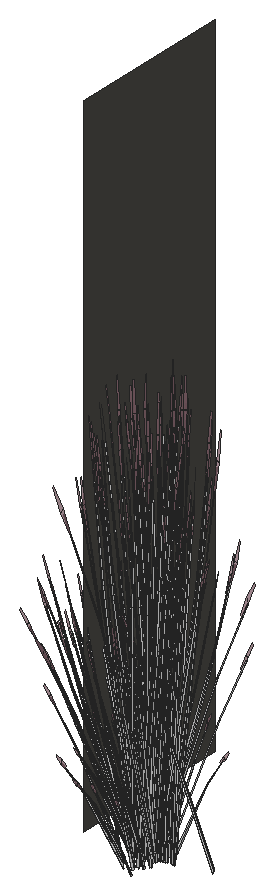
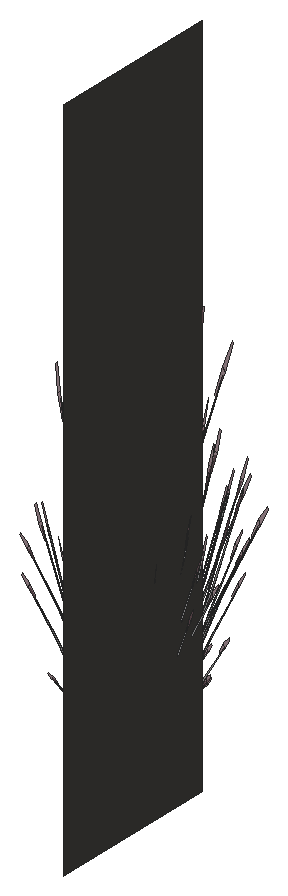
# SketchUp Ruby script. Lengths in inches.
U = 1.inch
M = Sketchup.active_model
def pt(a) = Geom::Point3d.new(a.map { |v| v * U })
def face(e, loops, mat)
  f = e.add_face(loops[0].map { |a| pt(a) })
  loops[1..].each { |l| e.add_face(l.map { |a| pt(a) }).erase! }
  f.material = f.back_material = mat if mat
  f
end
# faces: each face lists its corners as indices into pts; further lists are holes
def faces(e, pts, list, mat = nil) = list.each { |f| face(e, (f[0].is_a?(Array) ? f : [f]).map { |l| l.map { |i| pts[i] } }, mat) }
# xy, xz, yz: faces in a plane at the given z, y or x. An outline is a flat list of corners, or four numbers for a rectangle; further outlines are holes
def ring(l) = l.size == 4 ? [[l[0], l[1]], [l[2], l[1]], [l[2], l[3]], [l[0], l[3]]] : l.each_slice(2).to_a
def flat(e, list, mat, &to3) = list.each { |f| face(e, (f[0].is_a?(Array) ? f : [f]).map { |l| ring(l).map { |u, v| to3.(u, v) } }, mat) }
def xy(e, z, list, mat = nil) = flat(e, list, mat) { |x, y| [x, y, z] }
def xz(e, y, list, mat = nil) = flat(e, list, mat) { |x, z| [x, y, z] }
def yz(e, x, list, mat = nil) = flat(e, list, mat) { |y, z| [x, y, z] }
def lines(e, pts, list) = list.each { |a, b| e.add_line(pt(pts[a]), pt(pts[b])) }
# prism: a flat outline (further loops are holes) pulled along v
def prism(e, loops, v, mat = nil)
  f = face(e, loops, mat); d = Geom::Vector3d.new(v.map { |x| x * U })
  f.pushpull(f.normal.samedirection?(d) ? d.length : -d.length)
end
def box(e, o, s, mat = nil) = prism(e, [[o, [o[0] + s[0], o[1], o[2]], [o[0] + s[0], o[1] + s[1], o[2]], [o[0], o[1] + s[1], o[2]]]], [0, 0, s[2]], mat)
def at(x, y, z, deg = 0) = Geom::Transformation.translation(pt([x, y, z])) * Geom::Transformation.rotation(ORIGIN, Z_AXIS, deg.degrees)
def axes(o, x, y, z) = Geom::Transformation.new([*x, 0, *y, 0, *z, 0, *pt(o).to_a, 1])
def part(name) = M.definitions.add(name)
# library, detail: a bought-in or finely detailed component or shape, given as its bounding box
def library(name, o, s) = part(name).tap { |d| box(d.entities, o, s) }
def detail(e, o, s) = box(e.add_group.entities, o, s)
def put(e, d, t, mat = nil) = e.add_instance(d, t).tap { |i| i.material = mat if mat }
def group(e, t, mat = nil) = e.add_group.tap { |g| g.transformation = t; g.material = mat if mat }.entities
root = M.entities
M.materials.add("LightPink_Translucent").color = [144, 107, 117]
M.materials["LightPink_Translucent"].alpha = 0.75
M.materials.add("Wood_Planks_01_1K").color = [69, 67, 63]
M.materials.add("[_0053_Ivory_]").color = [200, 200, 200]
c1 = part("blade")
p = [[2.15,0.21,22],[0,0.17,0],[0.09,0.45,0],[2.18,0.31,22],[2.29,0.31,22],[0.38,0.45,0],
  [2.48,0.24,33],[2.49,0.24,33],[2.48,0.22,33]]
faces(c1.entities,p,[[0,1,2,3],[4,5,2,3],[6,3,4,7],[8,0,3,6]])
c2 = part("seeds")
p = [[0.3,-0.1,1.38],[-0.01,-0.03,1.59],[-0.01,-0.03,0.03],[0.14,-0.07,-0.07],[0.29,-0.03,3],[0.15,0.01,3.11]]
faces(c2.entities,p,[[0,1,2,3],[1,0,4,5]],"LightPink_Translucent")
c3 = part("blade with seeds")
put(c3.entities,c1,at(0,0,0))
put(c3.entities,c2,axes([2.4,0.25,30.99],[1.5799,-0.05474,1.17369],[-0.12525,1.92788,0.29478],[-0.07173,-0.02425,1.56792]))
yz(root,410.51,[[98.15,129,122.15,225]],"Wood_Planks_01_1K")
put(root,c3,axes([417.74,97.49,130.53],[0.25192,-0.01424,1.71376],[-0.16712,0.61729,0.13857],[-0.35901,-0.03818,0.73262]),"[_0053_Ivory_]")
put(root,c3,axes([417.85,98.57,130.53],[0.21074,-0.13302,1.71376],[0.17741,0.61464,0.13857],[-0.33083,0.13891,0.73262]),"[_0053_Ivory_]")
put(root,c3,axes([417.1875,99.62,129.24],[0.21107,0.05162,1.43002],[0.13604,0.52729,-0.30754],[-0.28671,0.0987,0.61141]),"[_0053_Ivory_]")
put(root,c3,axes([419.06,97.93,130],[0.17264,-0.09097,1.77064],[0.05953,0.63516,0.13857],[-0.37394,0.08428,0.63284]),"[_0053_Ivory_]")
put(root,c3,axes([418.49,96.91,131.63],[-0.60713,-0.01514,-0.71045],[0.04078,-0.63759,0.08574],[-0.25721,-0.06729,1.00501]),"[_0053_Ivory_]")
put(root,c3,axes([418,97.07,129.24],[0.11858,0.17508,1.43002],[-0.27325,0.4759,-0.30754],[-0.28057,-0.11375,0.61141]),"[_0053_Ivory_]")
put(root,c3,axes([417.52,98.02,131.18],[-0.50475,-0.17543,-0.35414],[0.14722,-0.5118,0.4572],[-0.20322,0.04693,0.87481]),"[_0053_Ivory_]")
put(root,c3,axes([418.22,96.5,130.53],[0.2256,0.10835,1.71376],[-0.46687,0.45453,0.13857],[-0.29098,-0.20505,0.73262]),"[_0053_Ivory_]")
put(root,c3,axes([417.87,98.28,131.33],[-0.16454,0.57202,-0.51099],[-0.56413,-0.19607,-0.3958],[-0.22713,0.05245,0.97773]),"[_0053_Ivory_]")
put(root,c3,axes([418.29,97.04,131.33],[-0.44101,0.41656,-0.51099],[-0.38623,-0.44004,-0.3958],[-0.22407,-0.06338,0.97773]),"[_0053_Ivory_]")
put(root,c3,axes([417.58,98.24,128.15],[0.0154,0.09911,1.76342],[-0.31051,0.51756,-0.26939],[-0.22056,-0.02609,0.30037]),"[_0053_Ivory_]")
put(root,c3,axes([416.75,100.73,129.42],[0.25312,-0.28501,1.1486],[0.09988,0.45119,0.84392],[-0.18292,0.08079,0.25299]),"[_0053_Ivory_]")
put(root,c3,axes([418.13,96.65,131.18],[-0.34557,-0.39372,-0.35414],[0.39459,-0.37271,0.4572],[-0.20048,-0.05671,0.87481]),"[_0053_Ivory_]")
put(root,c3,axes([418.62,98.99,130.53],[0.1517,-0.19322,1.71376],[0.38303,0.52154,0.13857],[-0.26271,0.23751,0.73262]),"[_0053_Ivory_]")
put(root,c3,axes([417.7,99.49,131.18],[-0.52868,0.08987,-0.35414],[-0.1396,-0.51376,0.4572],[-0.1515,0.13799,0.87481]),"[_0053_Ivory_]")
put(root,c3,axes([417.42,101.02,128.15],[0.08147,0.06283,1.76342],[0.13814,0.58211,-0.26939],[-0.18056,0.12413,0.30037]),"[_0053_Ivory_]")
put(root,c3,axes([417.3,97.59,129.42],[0.38775,-0.045,1.1486],[-0.24596,0.39648,0.84392],[-0.19161,-0.05948,0.25299]),"[_0053_Ivory_]")
put(root,c3,axes([418.5,99.46,130.53],[0.11309,-0.21615,1.71376],[0.47441,0.44731,0.13857],[-0.21402,0.27879,0.73262]),"[_0053_Ivory_]")
put(root,c3,axes([418.14,99.55,131.33],[0.15602,0.5742,-0.51099],[-0.59087,0.10045,-0.3958],[-0.16933,0.15423,0.97773]),"[_0053_Ivory_]")
put(root,c3,axes([419.61,99.14,128.71],[-0.63179,-0.1031,-0.62353],[0.13332,-0.63596,-0.16365],[-0.18854,-0.07706,1.37633]),"[_0053_Ivory_]")
put(root,c3,axes([419.55,96.16,131.63],[-0.51789,-0.30395,-0.71045],[0.36805,-0.53263,0.08574],[-0.18764,-0.18149,1.00501]),"[_0053_Ivory_]")
put(root,c3,axes([419.31,96.18,131.33],[-0.59932,0.14948,-0.51099],[-0.10484,-0.56611,-0.3958],[-0.16097,-0.16223,0.97773]),"[_0053_Ivory_]")
put(root,c3,axes([418.78,100.34,128.67],[-0.56842,-0.31443,-0.49651],[0.33976,-0.56381,0],[-0.12946,-0.07161,1.57504]),"[_0053_Ivory_]")
put(root,c3,axes([418.53,95.66,128.15],[-0.05883,0.08284,1.76342],[-0.59454,0.17861,-0.26939],[-0.14363,-0.16248,0.30037]),"[_0053_Ivory_]")
put(root,c3,axes([419.13,100.72,129.03],[-0.37973,0.63014,0],[-0.6353,-0.35142,-0.51607],[-0.14469,-0.08004,1.63711]),"[_0053_Ivory_]")
put(root,c3,axes([418.4375,101.64,129.24],[0.19166,-0.0992,1.43002],[0.4732,0.29912,-0.30754],[-0.14084,0.25882,0.61141]),"[_0053_Ivory_]")
put(root,c3,axes([418.17,95.98,128.78],[-0.1752,0.51349,-0.03893],[-0.53924,-0.15795,-0.17649],[-0.08187,-0.08399,0.58215]),"[_0053_Ivory_]")
put(root,c3,axes([418.97,95.33,129.24],[-0.03678,0.20572,1.43002],[-0.53767,0.17221,-0.30754],[-0.12568,-0.26589,0.61141]),"[_0053_Ivory_]")
put(root,c3,axes([419.15,95.87,130.53],[0.13883,0.2019,1.71376],[-0.64153,0.16998,0.13857],[-0.14499,-0.31697,0.73262]),"[_0053_Ivory_]")
put(root,c3,axes([420.33,99.24,129.32],[-0.61322,0.4175,-0.29095],[-0.40778,-0.58992,-0.50002],[-0.1513,-0.05991,1.59708]),"[_0053_Ivory_]")
put(root,c3,axes([419.37,95.76,131.18],[-0.0938,-0.50652,-0.35414],[0.53623,-0.13375,0.4572],[-0.14403,-0.14515,0.87481]),"[_0053_Ivory_]")
put(root,c3,axes([417.875,98.32,129.03],[-0.75945,0,0],[0,-0.70283,-0.51607],[0,-0.16007,1.63711]),"[_0053_Ivory_]")
put(root,c3,axes([418.94,100.11,128.68],[-0.14267,-0.54795,-0.30978],[0.56663,-0.1556,0.30978],[-0.11423,-0.06319,1.38974]),"[_0053_Ivory_]")
put(root,c3,axes([418.63,100.68,131.18],[-0.41095,0.33109,-0.35414],[-0.38901,-0.37805,0.4572],[-0.05919,0.19208,0.87481]),"[_0053_Ivory_]")
put(root,c3,axes([420.74,99.69,128.71],[-0.40909,0.47266,-0.62353],[-0.50819,-0.4286,-0.16365],[-0.16393,0.11791,1.37633]),"[_0053_Ivory_]")
put(root,c3,axes([418.46,98.14,128.98],[-0.56493,0.5287,0.30756],[-0.56528,-0.52313,-0.36492],[-0.01973,-0.15014,1.64885]),"[_0053_Ivory_]")
put(root,c3,axes([420.79,99.6,129.98],[0.52485,0.25358,1.51261],[-0.51417,0.54629,0.59816],[-0.23031,-0.32378,1.26806]),"[_0053_Ivory_]")
put(root,c3,axes([418.79,95,129.42],[0.31682,0.21887,1.1486],[-0.4614,0.13157,0.84392],[-0.09872,-0.16821,0.25299]),"[_0053_Ivory_]")
put(root,c3,axes([421.02,99.43,129.12],[-0.59306,-0.50614,-0.25192],[0.49904,-0.56836,0.5513],[-0.1597,0.05921,1.68216]),"[_0053_Ivory_]")
put(root,c3,axes([419.94,98.9375,128.86],[-0.36485,-0.52782,-0.44739],[0.55265,-0.37168,0.21531],[-0.11807,-0.06531,1.43643]),"[_0053_Ivory_]")
put(root,c3,axes([418.91,100.33,131.99],[-0.0158,0.58168,-0.7886],[-0.66548,-0.03907,0.09517],[-0.07023,0.24643,1.11556]),"[_0053_Ivory_]")
put(root,c3,axes([418.9,101.97,129.42],[-0.01572,-0.37392,1.1486],[0.39276,0.26669,0.84392],[-0.07724,0.17822,0.25299]),"[_0053_Ivory_]")
put(root,c3,axes([420.72,99.32,128.86],[-0.65953,0.03882,-0.44739],[-0.05964,-0.64439,0.21531],[-0.11807,0.06531,1.43643]),"[_0053_Ivory_]")
put(root,c3,axes([419.46,100.4,129.13],[0.56842,0.31443,0.49651],[-0.33976,0.56381,0],[-0.12946,-0.07161,1.57504]),"[_0053_Ivory_]")
put(root,c3,axes([418.69,101.15,130.02],[0.01334,-0.32463,1.54345],[0.60018,0.17147,0.21329],[-0.052,0.34598,0.72882]),"[_0053_Ivory_]")
put(root,c3,axes([419.99,99.24,129.09],[0.16098,-0.74515,-0.23429],[0.76326,0.12989,0.51271],[-0.13337,-0.1029,1.5644]),"[_0053_Ivory_]")
put(root,c3,axes([420.27,99.42,129.27],[-0.11717,0.56122,0.1448],[-0.57245,-0.09742,-0.41347],[-0.10418,-0.05763,1.26744]),"[_0053_Ivory_]")
put(root,c3,axes([421.41,100.98,128.67],[-0.56842,0.31443,-0.49651],[-0.33976,-0.56381,0],[-0.12946,0.07161,1.57504]),"[_0053_Ivory_]")
put(root,c3,axes([418.05,97.85,128.67],[0,-0.62885,-0.49651],[0.67951,0,0],[0,-0.14322,1.57504]),"[_0053_Ivory_]")
put(root,c3,axes([418.34,98.43,129.13],[0,0.62885,0.49651],[-0.67951,0,0],[0,-0.14322,1.57504]),"[_0053_Ivory_]")
put(root,c3,axes([421.45,100.8125,128.85],[-0.37499,-0.63235,-0.05142],[0.6353,-0.35142,0.51607],[-0.15655,0.0602,1.6363]),"[_0053_Ivory_]")
put(root,c3,axes([419.04,100.53,131.66],[0.43478,0.42253,-0.5672],[-0.45929,0.37004,-0.43934],[-0.06615,0.21468,1.08528]),"[_0053_Ivory_]")
put(root,c3,axes([421.28,100.73,128.68],[-0.56663,-0.1556,-0.30978],[0.14267,-0.54795,0.30978],[-0.11423,0.06319,1.38974]),"[_0053_Ivory_]")
put(root,c3,axes([419.82,98.58,129.32],[-0.68399,-0.30005,-0.29095],[0.32934,-0.63331,-0.50002],[-0.0215,-0.15549,1.59708]),"[_0053_Ivory_]")
put(root,c3,axes([421.6,98.39,129.5],[-0.01659,-0.59209,1.41272],[0.75089,0.15348,0.59816],[-0.1776,0.32398,1.3335]),"[_0053_Ivory_]")
put(root,c3,axes([418.57,101.16,129.48],[0.55175,-0.11136,0.06507],[0.12684,0.44864,-0.86304],[-0.03498,0.22711,0.7736]),"[_0053_Ivory_]")
put(root,c3,axes([421.18,99.14,129.32],[0.07077,0.71755,-0.29095],[-0.73712,0.04339,-0.50002],[-0.1298,0.09558,1.59708]),"[_0053_Ivory_]")
put(root,c3,axes([419.52,97.9375,128.75],[-0.24943,-0.64486,-0.69835],[0.71849,-0.23224,-0.18329],[-0.02757,-0.21836,1.54149]),"[_0053_Ivory_]")
put(root,c3,axes([420.64,95.91,131.33],[-0.59704,-0.15764,-0.51099],[0.20464,-0.54049,-0.3958],[-0.05475,-0.21761,0.97773]),"[_0053_Ivory_]")
put(root,c3,axes([419.54,99.92,130.53],[-0.01487,-0.24136,1.71376],[0.64429,0.16012,0.13857],[-0.03985,0.34396,0.73262]),"[_0053_Ivory_]")
put(root,c3,axes([418.34,97.86,128.68],[0.42396,-0.39235,-0.30978],[0.42396,0.39235,0.30978],[0,-0.12637,1.38974]),"[_0053_Ivory_]")
put(root,c3,axes([420.25,95.32,128.78],[-0.4197,0.36076,-0.03893],[-0.38456,-0.39511,-0.17649],[-0.02707,-0.11196,0.58215]),"[_0053_Ivory_]")
put(root,c3,axes([420.08,98.88,129.01],[0.76764,0.13249,0.45755],[-0.15622,0.74829,0.17955],[-0.11218,-0.07226,1.58856]),"[_0053_Ivory_]")
put(root,c3,axes([419.88,98.75,129.37],[-0.29468,0.56664,0.44739],[-0.61229,-0.27271,-0.21531],[0,-0.13062,1.43643]),"[_0053_Ivory_]")
put(root,c3,axes([420.86,96.02,131.63],[-0.28988,-0.51132,-0.71045],[0.59671,-0.28496,0.08574],[-0.06778,-0.24706,1.00501]),"[_0053_Ivory_]")
put(root,c3,axes([419.67,100.08,129.13],[0.65264,-0.16691,0.17642],[0.16115,0.62115,0.35086],[-0.05821,-0.0905,1.60407]),"[_0053_Ivory_]")
put(root,c3,axes([420.51,100.18,128.85],[-0.61229,-0.28233,0],[0.29468,-0.58663,0],[0,0,1.62707]),"[_0053_Ivory_]")
put(root,c3,axes([421.93,100.88,129.03],[0.37973,0.63014,0],[-0.6353,0.35142,-0.51607],[-0.14469,0.08004,1.63711]),"[_0053_Ivory_]")
put(root,c3,axes([421.61,100.11,129.13],[0.17545,-0.62497,0.17642],[0.64204,0.17686,0.35086],[-0.11091,0.00304,1.60407]),"[_0053_Ivory_]")
put(root,c3,axes([421.32,99.28,129.27],[0.44871,0.37783,0.1448],[-0.37428,0.42627,-0.41347],[-0.10418,0.05763,1.26744]),"[_0053_Ivory_]")
put(root,c3,axes([421.16,98.82,128.95],[-0.56493,-0.54126,-0.06131],[0.56528,-0.54159,0],[-0.01973,-0.0189,1.75571]),"[_0053_Ivory_]")
put(root,c3,axes([421.3,99.01,129.37],[0.65953,-0.03882,0.44739],[0.05964,0.64439,-0.21531],[-0.11807,0.06531,1.43643]),"[_0053_Ivory_]")
put(root,c3,axes([421.47,100.49,128.98],[0.76036,0.2044,0.30756],[-0.19023,0.7306,-0.36492],[-0.12585,0.09144,1.64885]),"[_0053_Ivory_]")
put(root,c3,axes([420.36,94.88,128.15],[-0.10187,0.02266,1.76342],[-0.56336,-0.25503,-0.26939],[0.00945,-0.21273,0.30037]),"[_0053_Ivory_]")
put(root,c3,axes([421.79,100.45,129.13],[0.56842,-0.31443,0.49651],[0.33976,0.56381,0],[-0.12946,0.07161,1.57504]),"[_0053_Ivory_]")
put(root,c3,axes([420.91,95.58,131.18],[0.1831,-0.48359,-0.35414],[0.53419,0.14105,0.4572],[-0.04898,-0.1947,0.87481]),"[_0053_Ivory_]")
put(root,c3,axes([420.02,98.19,129.01],[0.26406,0.70318,0.45755],[-0.7545,0.24452,0.17955],[0.00922,-0.12921,1.58856]),"[_0053_Ivory_]")
put(root,c3,axes([419.89,98.1,128.86],[0.29468,-0.56664,-0.44739],[0.61229,0.27271,0.21531],[0,-0.13062,1.43643]),"[_0053_Ivory_]")
put(root,c3,axes([420.65,99.93,128.86],[-0.19817,-0.54216,0],[0.56587,-0.18986,0],[0,0,1.54371]),"[_0053_Ivory_]")
put(root,c3,axes([419.93,101.08,128.15],[0.09829,-0.03422,1.76342],[0.59126,0.18834,-0.26939],[0.01729,0.21228,0.30037]),"[_0053_Ivory_]")
put(root,c3,axes([420.06,101.27,131.18],[-0.1831,0.48359,-0.35414],[-0.53419,-0.14105,0.4572],[0.04898,0.1947,0.87481]),"[_0053_Ivory_]")
put(root,c3,axes([421.45,98.86,128.86],[-0.29468,0.56664,-0.44739],[-0.61229,-0.27271,0.21531],[0,0.13062,1.43643]),"[_0053_Ivory_]")
put(root,c3,axes([422.61,98.52,129.13],[-0.47719,-0.45806,0.17642],[0.48088,-0.44429,0.35086],[-0.0527,0.09355,1.60407]),"[_0053_Ivory_]")
put(root,c3,axes([420.97,98.25,128.86],[0,-0.72763,0],[0.75945,0,0],[0,0,1.79456]),"[_0053_Ivory_]")
put(root,c3,axes([420.26,98.39,129.09],[0.68433,0.30479,0.24065],[-0.32934,0.63331,0.50002],[0,-0.14599,1.60543]),"[_0053_Ivory_]")
put(root,c3,axes([421.35,98.54,128.95],[0,0.72727,-0.05637],[-0.75945,0,0],[0,0.02286,1.79368]),"[_0053_Ivory_]")
put(root,c3,axes([420.04,97.96,129.37],[-0.65953,0.03882,0.44739],[-0.05964,-0.64439,-0.21531],[0.11807,-0.06531,1.43643]),"[_0053_Ivory_]")
put(root,c3,axes([419.73,96.85,129.13],[-0.17545,0.62497,0.17642],[-0.64204,-0.17686,0.35086],[0.11091,-0.00304,1.60407]),"[_0053_Ivory_]")
put(root,c3,axes([420.98,99.95,128.94],[0.26406,0.72244,-0.06012],[-0.7545,0.25315,0],[0.00922,0.02523,1.72173]),"[_0053_Ivory_]")
put(root,c3,axes([419.42,96.08,129.03],[-0.37973,-0.63014,0],[0.6353,-0.35142,-0.51607],[0.14469,-0.08004,1.63711]),"[_0053_Ivory_]")
put(root,c3,axes([420.12,100.83,131.63],[0.28988,0.51132,-0.71045],[-0.59671,0.28496,0.08574],[0.06778,0.24706,1.00501]),"[_0053_Ivory_]")
put(root,c3,axes([423.17,99,128.85],[-0.75908,-0.00503,-0.04976],[0,-0.70283,0.49943],[-0.02386,0.16,1.58352]),"[_0053_Ivory_]")
put(root,c3,axes([421.67,96.89,129.13],[-0.65264,0.16691,0.17642],[-0.16115,-0.62115,0.35086],[0.05821,0.0905,1.60407]),"[_0053_Ivory_]")
put(root,c3,axes([421.01,94.5625,129.42],[0.07791,0.3667,1.1486],[-0.43222,-0.2031,0.84392],[0.04651,-0.18776,0.25299]),"[_0053_Ivory_]")
put(root,c3,axes([420.61,97.79,129.01],[-0.50358,0.57069,0.45755],[-0.59827,-0.50377,0.17955],[0.1214,-0.05695,1.58856]),"[_0053_Ivory_]")
put(root,c3,axes([421.47,98.69,128.87],[0.42396,0.40619,0],[-0.42396,0.40619,0],[0,0,1.69266]),"[_0053_Ivory_]")
put(root,c3,axes([421.46,98.22,129.37],[0.29468,-0.56664,0.44739],[0.61229,0.27271,-0.21531],[0,0.13062,1.43643]),"[_0053_Ivory_]")
put(root,c3,axes([421.2,100.1875,128.86],[0.61229,0.28233,0],[-0.29468,0.58663,0],[0,0,1.74954]),"[_0053_Ivory_]")
put(root,c3,axes([420.33,100.94,131.33],[0.59704,0.15764,-0.51099],[-0.20464,0.54049,-0.3958],[0.05475,0.21761,0.97773]),"[_0053_Ivory_]")
put(root,c3,axes([421.26,98.08,129.03],[-0.76764,-0.13249,0.49198],[0.15622,-0.74829,0.19306],[0.11218,0.07226,1.70813]),"[_0053_Ivory_]")
put(root,c3,axes([423.01,99.11,128.68],[-0.42396,0.39235,-0.30978],[-0.42396,-0.39235,0.30978],[0,0.12637,1.38974]),"[_0053_Ivory_]")
put(root,c3,axes([421.8,99.03,128.75],[0.2227,0.57576,-0.69212],[-0.64151,0.20736,-0.18165],[0.02462,0.19497,1.52773]),"[_0053_Ivory_]")
put(root,c3,axes([421.48,98.42,128.86],[0.67951,0,0],[0,0.65103,0],[0,0,1.78407]),"[_0053_Ivory_]")
put(root,c3,axes([420.83,97.7,129.37],[-0.36485,-0.52782,0.44739],[0.55265,-0.37168,-0.21531],[0.11807,0.06531,1.43643]),"[_0053_Ivory_]")
put(root,c3,axes([420.16,97.82,129.32],[-0.07077,-0.71755,-0.29095],[0.73712,-0.04339,-0.50002],[0.1298,-0.09558,1.59708]),"[_0053_Ivory_]")
put(root,c3,axes([421.72,98.35,129.27],[0.56587,-0.18339,0.1448],[0.19817,0.52368,-0.41347],[0,0.11525,1.26744]),"[_0053_Ivory_]")
put(root,c3,axes([421.93,96.32,131.33],[-0.43478,-0.42253,-0.51099],[0.45929,-0.37004,-0.3958],[0.06615,-0.21468,0.97773]),"[_0053_Ivory_]")
put(root,c3,axes([421.52,98.39,129.32],[0.68399,0.30005,-0.29095],[-0.32934,0.63331,-0.50002],[0.0215,0.15549,1.59708]),"[_0053_Ivory_]")
put(root,c3,axes([420.07,96.23,128.68],[0.56663,0.1556,-0.30978],[-0.14267,0.54795,0.30978],[0.11423,-0.06319,1.38974]),"[_0053_Ivory_]")
put(root,c3,axes([421.64,95.57,129.24],[-0.17264,0.12729,1.43002],[-0.51703,-0.22279,-0.30754],[0.09584,-0.27707,0.61141]),"[_0053_Ivory_]")
put(root,c3,axes([423.01,98.54,129.13],[0,-0.62885,0.49651],[0.67951,0,0],[0,0.14322,1.57504]),"[_0053_Ivory_]")
put(root,c3,axes([423.3,99.12,128.67],[0,0.62885,-0.49651],[-0.67951,0,0],[0,0.14322,1.57504]),"[_0053_Ivory_]")
put(root,c3,axes([419.93,95.99,128.67],[0.56842,-0.31443,-0.49651],[0.33976,0.56381,0],[0.12946,-0.07161,1.57504]),"[_0053_Ivory_]")
put(root,c3,axes([420.67,99.82,130.53],[-0.13883,-0.2019,1.71376],[0.64153,-0.16998,0.13857],[0.14499,0.31697,0.73262]),"[_0053_Ivory_]")
put(root,c3,axes([421.07,97.55,129.27],[0.11717,-0.56122,0.1448],[0.57245,0.09742,-0.41347],[0.10418,0.05763,1.26744]),"[_0053_Ivory_]")
put(root,c3,axes([421.89,96.57,129.13],[-0.56842,-0.31443,0.49651],[0.33976,-0.56381,0],[0.12946,0.07161,1.57504]),"[_0053_Ivory_]")
put(root,c3,axes([422.0625,96.52,131.63],[0.0158,-0.58168,-0.71045],[0.66548,0.03907,0.08574],[0.07023,-0.24643,1.00501]),"[_0053_Ivory_]")
put(root,c3,axes([421.39,99.86,128.84],[0.63764,-0.21337,-0.19198],[0.22406,0.61462,0.00008],[0.07038,-0.02358,1.73897]),"[_0053_Ivory_]")
put(root,c3,axes([429.95,97.49,130.53],[0.25192,-0.01424,1.71376],[-0.16712,0.61729,0.13857],[-0.35901,-0.03818,0.73262]),"[_0053_Ivory_]")
put(root,c3,axes([421.4,98.03,128.86],[0.36485,0.52782,-0.44739],[-0.55265,0.37168,0.21531],[0.11807,0.06531,1.43643]),"[_0053_Ivory_]")
put(root,c3,axes([422.34,96.17,131.18],[0.41095,-0.33109,-0.35414],[0.38901,0.37805,0.4572],[0.05919,-0.19208,0.87481]),"[_0053_Ivory_]")
put(root,c3,axes([422.4375,100.42,129.42],[-0.34197,-0.18082,1.1486],[0.44156,-0.18372,0.84392],[0.1191,0.15563,0.25299]),"[_0053_Ivory_]")
put(root,c3,axes([421.22,100.23,129.24],[0.01072,-0.20846,1.43002],[0.51218,-0.23285,-0.30754],[0.15811,0.2495,0.61141]),"[_0053_Ivory_]")
put(root,c3,axes([420.61,97.28,128.71],[0.40909,-0.47266,-0.62353],[0.50819,0.4286,-0.16365],[0.16393,-0.11791,1.37633]),"[_0053_Ivory_]")
